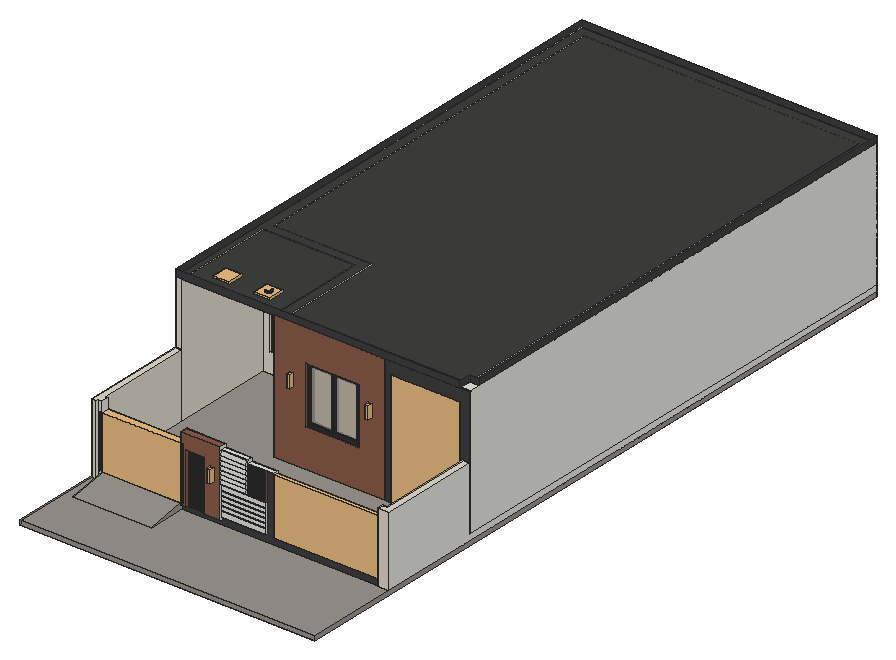
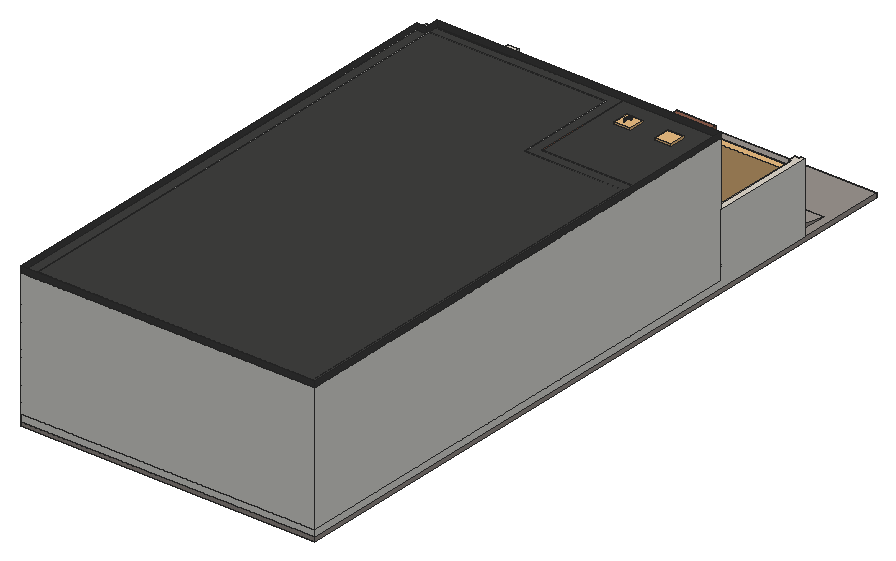
# SketchUp Ruby script. Lengths in inches.
U = 1.inch
M = Sketchup.active_model
def pt(a) = Geom::Point3d.new(a.map { |v| v * U })
def face(e, loops, mat)
  f = e.add_face(loops[0].map { |a| pt(a) })
  loops[1..].each { |l| e.add_face(l.map { |a| pt(a) }).erase! }
  f.material = f.back_material = mat if mat
  f
end
# faces: each face lists its corners as indices into pts; further lists are holes
def faces(e, pts, list, mat = nil) = list.each { |f| face(e, (f[0].is_a?(Array) ? f : [f]).map { |l| l.map { |i| pts[i] } }, mat) }
# xy, xz, yz: faces in a plane at the given z, y or x. An outline is a flat list of corners, or four numbers for a rectangle; further outlines are holes
def ring(l) = l.size == 4 ? [[l[0], l[1]], [l[2], l[1]], [l[2], l[3]], [l[0], l[3]]] : l.each_slice(2).to_a
def flat(e, list, mat, &to3) = list.each { |f| face(e, (f[0].is_a?(Array) ? f : [f]).map { |l| ring(l).map { |u, v| to3.(u, v) } }, mat) }
def xy(e, z, list, mat = nil) = flat(e, list, mat) { |x, y| [x, y, z] }
def xz(e, y, list, mat = nil) = flat(e, list, mat) { |x, z| [x, y, z] }
def yz(e, x, list, mat = nil) = flat(e, list, mat) { |y, z| [x, y, z] }
def lines(e, pts, list) = list.each { |a, b| e.add_line(pt(pts[a]), pt(pts[b])) }
# prism: a flat outline (further loops are holes) pulled along v
def prism(e, loops, v, mat = nil)
  f = face(e, loops, mat); d = Geom::Vector3d.new(v.map { |x| x * U })
  f.pushpull(f.normal.samedirection?(d) ? d.length : -d.length)
end
def box(e, o, s, mat = nil) = prism(e, [[o, [o[0] + s[0], o[1], o[2]], [o[0] + s[0], o[1] + s[1], o[2]], [o[0], o[1] + s[1], o[2]]]], [0, 0, s[2]], mat)
def at(x, y, z, deg = 0) = Geom::Transformation.translation(pt([x, y, z])) * Geom::Transformation.rotation(ORIGIN, Z_AXIS, deg.degrees)
def axes(o, x, y, z) = Geom::Transformation.new([*x, 0, *y, 0, *z, 0, *pt(o).to_a, 1])
def part(name) = M.definitions.add(name)
# library, detail: a bought-in or finely detailed component or shape, given as its bounding box
def library(name, o, s) = part(name).tap { |d| box(d.entities, o, s) }
def detail(e, o, s) = box(e.add_group.entities, o, s)
def put(e, d, t, mat = nil) = e.add_instance(d, t).tap { |i| i.material = mat if mat }
def group(e, t, mat = nil) = e.add_group.tap { |g| g.transformation = t; g.material = mat if mat }.entities
root = M.entities
M.materials.add("1448 AP 8253 RAVEN SONG").color = [64, 64, 63]
M.materials.add("[Chris_Hair]").color = [71, 76, 74]
M.materials.add("[Granite Tile]").color = [155, 148, 143]
M.materials.add("[Steel Brushed Stainless]").color = [51, 51, 51]
M.materials.add("[Stone Vein Gray]").color = [63, 63, 63]
M.materials.add("[Tile Various Tan]").color = [223, 216, 204]
M.materials.add("[Translucent Glass Gray]").color = [181, 181, 181]
M.materials["[Translucent Glass Gray]"].alpha = 0.5
M.materials.add("[Wax 02]").color = [139, 92, 74]
M.materials.add("[Wood Veneer 01]").color = [91, 58, 35]
c1 = part("8")
box(c1.entities,[0,0.25,0],[0.5,0.25,24.5])
c2 = part("9")
box(c2.entities,[0,0,0],[0.25,0.25,48.1875])
c3 = library("Group\#151",[0,0,0],[124.17,4.81,62])
c4 = library("Curtains",[0,0,0],[121.73,8.19,117.22])
c5 = library("porte moderne noir",[57.21,0.32,0],[43.81,4.72,87.03])
c6 = part("Group\#3")
g1 = group(c6.entities,at(0,3,0))
prism(g1,[[[9,0,0],[0,0,0],[0,0,72],[9,0,72]],[[0.75,0,71.25],[0.75,0,0.75],[8.25,0,0.75],[8.25,0,71.25]]],[0,-1,0])
g2 = group(g1,at(0.75,-0.26,0.75),"[Translucent Glass Gray]")
box(g2,[0,-0.47,0],[7.5,0.47,70.5])
c7 = part("Group\#8")
g3 = group(c7.entities,at(0,1.75,0))
prism(g3,[[[21,0,0],[0,0,0],[0,0,50],[21,0,50]],[[20,0,49],[1,0,49],[1,0,1],[20,0,1]]],[0,-1.5,0])
g4 = group(g3,at(1,-0.5,1),"[Translucent Glass Gray]")
box(g4,[0,-0.47,0],[19,0.47,48])
c8 = library("Group\#93",[0,-4.51,0],[63,7.09,108])
c9 = library("Component",[1.03,-1.63,0],[72.41,6.81,50.39])
c10 = library("WALL LIGHT 69",[4.19,4.05,-8.78],[4.61,5.7,17.13])
c11 = library("11",[-5.64,-5.64,-13.23],[15.28,15.28,13.23])
xy(root,120,[[[9.27,183,9.27,663,287.37,663,287.37,195,278.1,195,278.1,183],[39.35,204,39.59,204,39.66,204.01,39.74,204.01,39.9,204.03,39.98,204.05,40.05,204.0625,40.13,204.08,40.21,204.1,40.28,204.12,40.36,204.14,40.43,204.17,40.51,204.19,40.72,204.28,40.79,204.32,40.86,204.35,41.07,204.47,41.13,204.52,41.2,204.5625,41.26,204.61,41.56,204.86,41.61,204.92,41.67,204.98,41.82,205.16,41.86,205.22,41.91,205.28,41.95,205.35,42,205.42,42.04,205.48,42.08,205.55,42.11,205.62,42.15,205.69,42.21,205.83,42.24,205.91,42.3,206.05,42.32,206.13,42.34,206.2,42.38,206.36,42.4,206.43,42.43,206.67,42.4375,206.74,42.44,206.82,42.45,206.9,42.45,207.14,42.44,207.21,42.4375,207.29,42.43,207.37,42.42,207.45,42.4,207.53,42.39,207.6,42.35,207.76,42.33,207.83,42.31,207.91,42.28,207.98,42.26,208.06,42.17,208.27,42.13,208.34,42.1,208.41,41.98,208.62,41.93,208.68,41.89,208.75,41.59,209.11,41.53,209.16,41.47,209.22,41.29,209.37,41.23,209.41,41.17,209.46,41.1,209.5,41.03,209.55,40.97,209.59,40.83,209.66,40.76,209.7,40.6875,209.73,40.62,209.76,40.54,209.79,40.4,209.85,40.32,209.87,40.25,209.89,40.09,209.93,40.02,209.95,39.78,209.98,39.71,209.99,39.63,209.99,39.55,210,39.3125,210,39.24,209.99,39.16,209.99,39,209.97,38.92,209.95,38.85,209.9375,38.77,209.92,38.69,209.9,38.62,209.88,38.54,209.86,38.47,209.83,38.39,209.81,38.18,209.72,38.11,209.68,38.04,209.65,37.83,209.53,37.77,209.48,37.7,209.4375,37.64,209.39,37.34,209.14,37.29,209.08,37.23,209.02,37.08,208.84,37.04,208.78,36.99,208.72,36.95,208.65,36.9,208.58,36.86,208.52,36.82,208.45,36.79,208.38,36.75,208.31,36.72,208.24,36.6875,208.17,36.66,208.09,36.6,207.95,36.58,207.87,36.56,207.8,36.52,207.64,36.5,207.57,36.47,207.33,36.46,207.26,36.46,207.18,36.45,207.1,36.45,206.86,36.46,206.79,36.46,206.71,36.48,206.55,36.5,206.47,36.51,206.4,36.55,206.24,36.57,206.17,36.59,206.09,36.62,206.02,36.64,205.94,36.73,205.73,36.77,205.66,36.8,205.59,36.92,205.38,36.97,205.32,37.01,205.25,37.26,204.95,37.3125,204.89,37.37,204.84,37.43,204.78,37.61,204.63,37.67,204.59,37.73,204.54,37.8,204.5,37.87,204.45,37.93,204.41,38.07,204.34,38.14,204.3,38.28,204.24,38.36,204.21,38.5,204.15,38.58,204.13,38.65,204.11,38.81,204.07,38.88,204.05,39.12,204.02,39.19,204.01,39.27,204.01],[77.87,204,78.11,204,78.18,204.01,78.26,204.01,78.42,204.03,78.5,204.05,78.57,204.0625,78.65,204.08,78.73,204.1,78.8,204.12,78.88,204.14,78.95,204.17,79.03,204.19,79.24,204.28,79.3125,204.32,79.38,204.35,79.59,204.47,79.65,204.52,79.72,204.5625,79.78,204.61,80.08,204.86,80.13,204.92,80.1875,204.98,80.24,205.04,80.34,205.16,80.38,205.22,80.43,205.28,80.47,205.35,80.52,205.42,80.56,205.48,80.6,205.55,80.63,205.62,80.67,205.69,80.73,205.83,80.76,205.91,80.82,206.05,80.84,206.13,80.86,206.2,80.9,206.36,80.92,206.43,80.95,206.67,80.96,206.74,80.96,206.82,80.97,206.9,80.97,207.14,80.96,207.21,80.96,207.29,80.95,207.37,80.9375,207.45,80.92,207.53,80.91,207.6,80.89,207.68,80.875,207.76,80.85,207.83,80.83,207.91,80.8,207.98,80.78,208.06,80.72,208.2,80.6875,208.27,80.65,208.34,80.62,208.41,80.5,208.62,80.45,208.68,80.41,208.75,80.36,208.81,80.3125,208.87,80.26,208.93,80.11,209.11,80.05,209.16,79.99,209.22,79.93,209.27,79.875,209.32,79.8125,209.37,79.75,209.41,79.6875,209.46,79.62,209.5,79.55,209.55,79.49,209.59,79.35,209.66,79.28,209.7,79.14,209.76,79.0625,209.79,78.99,209.82,78.92,209.85,78.84,209.87,78.77,209.89,78.61,209.93,78.54,209.95,78.3,209.98,78.23,209.99,78.15,209.99,78.07,210,77.83,210,77.76,209.99,77.68,209.99,77.52,209.97,77.44,209.95,77.37,209.9375,77.29,209.92,77.21,209.9,77.14,209.88,77.0625,209.86,76.99,209.83,76.91,209.81,76.7,209.72,76.625,209.68,76.56,209.65,76.35,209.53,76.29,209.48,76.22,209.4375,76.16,209.39,75.86,209.14,75.81,209.08,75.75,209.02,75.6,208.84,75.56,208.78,75.51,208.72,75.47,208.65,75.42,208.58,75.38,208.52,75.34,208.45,75.31,208.38,75.27,208.31,75.21,208.17,75.18,208.09,75.15,208.02,75.125,207.95,75.1,207.87,75.08,207.8,75.04,207.64,75.02,207.57,74.99,207.33,74.98,207.26,74.98,207.18,74.97,207.1,74.97,206.86,74.98,206.79,74.98,206.71,75,206.55,75.02,206.47,75.03,206.4,75.07,206.24,75.09,206.17,75.11,206.09,75.14,206.02,75.16,205.94,75.25,205.73,75.29,205.66,75.32,205.59,75.44,205.38,75.49,205.32,75.53,205.25,75.58,205.19,75.625,205.13,75.68,205.07,75.83,204.89,75.89,204.84,75.95,204.78,76.13,204.63,76.19,204.59,76.25,204.54,76.32,204.5,76.39,204.45,76.45,204.41,76.59,204.34,76.66,204.3,76.8,204.24,76.95,204.18,77.02,204.15,77.1,204.13,77.17,204.11,77.33,204.07,77.4,204.05,77.64,204.02,77.71,204.01,77.79,204.01]]],"1448 AP 8253 RAVEN SONG")
xz(root,183,[[9.27,120,278.1,126]],"1448 AP 8253 RAVEN SONG")
xz(root,195,[[278.1,120,287.37,126]],"1448 AP 8253 RAVEN SONG")
xz(root,204,[[77.87,120,77.95,123],[77.95,120,78.03,123],[78.03,120,78.11,123]],"1448 AP 8253 RAVEN SONG")
xz(root,204.01,[[77.71,120,77.79,123],[78.18,120,78.26,123]],"1448 AP 8253 RAVEN SONG")
xz(root,663,[[9.27,120,287.37,126]],"1448 AP 8253 RAVEN SONG")
yz(root,9.27,[[183,120,663,126]],"1448 AP 8253 RAVEN SONG")
yz(root,80.96,[[206.74,120,206.82,123],[207.21,120,207.29,123]],"1448 AP 8253 RAVEN SONG")
yz(root,80.97,[[206.9,120,206.98,123],[206.98,120,207.06,123],[207.06,120,207.14,123]],"1448 AP 8253 RAVEN SONG")
yz(root,278.1,[[183,120,195,126]],"1448 AP 8253 RAVEN SONG")
yz(root,287.37,[[195,120,663,126]],"1448 AP 8253 RAVEN SONG")
p = [[77.48,204.04,120],[77.4,204.05,120],[77.4,204.05,123],[77.48,204.04,123],[77.56,204.03,120],[77.56,204.03,123],
  [77.71,204.01,120],[77.64,204.02,120],[77.64,204.02,123],[77.71,204.01,123],[77.87,204,120],[77.79,204.01,120],
  [77.79,204.01,123],[77.87,204,123],[78.18,204.01,120],[78.11,204,120],[78.11,204,123],[78.18,204.01,123],
  [78.42,204.03,120],[78.34,204.02,120],[78.34,204.02,123],[78.42,204.03,123],[78.26,204.01,120],[78.26,204.01,123],
  [78.5,204.05,120],[78.5,204.05,123],[78.57,204.0625,120],[78.57,204.0625,123],[77.1,204.13,120],[77.02,204.15,120],
  [77.02,204.15,123],[77.1,204.13,123],[77.17,204.11,120],[77.17,204.11,123],[77.33,204.07,120],[77.25,204.09,120],
  [77.25,204.09,123],[77.33,204.07,123],[78.65,204.08,120],[78.65,204.08,123],[78.8,204.12,120],[78.73,204.1,120],
  [78.73,204.1,123],[78.8,204.12,123],[78.88,204.14,120],[78.88,204.14,123],[78.95,204.17,120],[78.95,204.17,123],
  [76.875,204.21,120],[76.8,204.24,120],[76.8,204.24,123],[76.875,204.21,123],[76.95,204.18,120],[76.95,204.18,123],
  [79.1,204.22,120],[79.03,204.19,120],[79.03,204.19,123],[79.1,204.22,123],[79.17,204.25,120],[79.17,204.25,123],
  [79.3125,204.32,120],[79.24,204.28,120],[79.24,204.28,123],[79.3125,204.32,123],[79.38,204.35,120],[79.38,204.35,123],
  [79.45,204.39,120],[79.45,204.39,123],[79.59,204.47,120],[79.52,204.43,120],[79.52,204.43,123],[79.59,204.47,123],
  [79.65,204.52,120],[79.65,204.52,123],[79.72,204.5625,120],[79.72,204.5625,123],[79.78,204.61,120],[79.78,204.61,123],
  [79.84,204.66,120],[79.84,204.66,123],[79.9,204.71,120],[79.9,204.71,123],[79.96,204.76,120],[79.96,204.76,123],
  [80.08,204.86,120],[80.02,204.81,120],[80.02,204.81,123],[80.08,204.86,123],[80.1875,204.98,120],[80.13,204.92,120],
  [80.13,204.92,123],[80.1875,204.98,123],[80.29,205.1,120],[80.24,205.04,120],[80.24,205.04,123],[80.29,205.1,123],
  [80.34,205.16,120],[80.34,205.16,123],[80.38,205.22,120],[80.38,205.22,123],[80.43,205.28,120],[80.43,205.28,123],
  [80.47,205.35,120],[80.47,205.35,123],[80.52,205.42,120],[80.52,205.42,123],[80.56,205.48,120],[80.56,205.48,123],
  [80.6,205.55,120],[80.6,205.55,123],[80.67,205.69,120],[80.63,205.62,120],[80.63,205.62,123],[80.67,205.69,123],
  [80.7,205.76,120],[80.7,205.76,123],[80.76,205.91,120],[80.73,205.83,120],[80.73,205.83,123],[80.76,205.91,123],
  [80.79,205.98,120],[80.79,205.98,123],[80.82,206.05,120],[80.82,206.05,123],[80.86,206.2,120],[80.84,206.13,120],
  [80.84,206.13,123],[80.86,206.2,123],[80.88,206.28,120],[80.88,206.28,123],[80.9,206.36,120],[80.9,206.36,123],
  [80.93,206.51,120],[80.92,206.43,120],[80.92,206.43,123],[80.93,206.51,123],[80.94,206.59,120],[80.94,206.59,123],
  [80.95,206.67,120],[80.95,206.67,123],[80.96,206.74,120],[80.96,206.74,123],[80.97,206.9,120],[80.96,206.82,120],
  [80.96,206.82,123],[80.97,206.9,123],[80.96,207.21,120],[80.97,207.14,120],[80.97,207.14,123],[80.96,207.21,123],
  [80.95,207.37,120],[80.96,207.29,120],[80.96,207.29,123],[80.95,207.37,123],[80.92,207.53,120],[80.9375,207.45,120],
  [80.9375,207.45,123],[80.92,207.53,123],[80.91,207.6,120],[80.91,207.6,123],[80.89,207.68,120],[80.89,207.68,123],
  [80.875,207.76,120],[80.875,207.76,123],[80.83,207.91,120],[80.85,207.83,120],[80.85,207.83,123],[80.83,207.91,123],
  [80.8,207.98,120],[80.8,207.98,123],[80.78,208.06,120],[80.78,208.06,123],[80.72,208.2,120],[80.75,208.13,120],
  [80.75,208.13,123],[80.72,208.2,123],[80.6875,208.27,120],[80.6875,208.27,123],[80.62,208.41,120],[80.65,208.34,120],
  [80.65,208.34,123],[80.62,208.41,123],[80.58,208.48,120],[80.58,208.48,123],[80.5,208.62,120],[80.54,208.55,120],
  [80.54,208.55,123],[80.5,208.62,123],[80.45,208.68,120],[80.45,208.68,123],[80.36,208.81,120],[80.41,208.75,120],
  [80.41,208.75,123],[80.36,208.81,123],[80.3125,208.87,120],[80.3125,208.87,123],[80.21,208.99,120],[80.26,208.93,120],
  [80.26,208.93,123],[80.21,208.99,123],[80.16,209.05,120],[80.16,209.05,123],[80.05,209.16,120],[80.11,209.11,120],
  [80.11,209.11,123],[80.05,209.16,123],[79.93,209.27,120],[79.99,209.22,120],[79.99,209.22,123],[79.93,209.27,123],
  [79.8125,209.37,120],[79.875,209.32,120],[79.875,209.32,123],[79.8125,209.37,123],[79.75,209.41,120],[79.75,209.41,123]]
faces(root,p,[[0,1,2,3],[4,0,3,5],[6,7,8,9],[7,4,5,8],[10,11,12,13],[14,15,16,17],[18,19,20,21],[19,22,23,20],
  [24,18,21,25],[26,24,25,27],[28,29,30,31],[32,28,31,33],[34,35,36,37],[35,32,33,36],[1,34,37,2],[38,26,27,39],
  [40,41,42,43],[41,38,39,42],[44,40,43,45],[46,44,45,47],[48,49,50,51],[29,52,53,30],[52,48,51,53],[54,55,56,57],
  [55,46,47,56],[58,54,57,59],[60,61,62,63],[61,58,59,62],[64,60,63,65],[66,64,65,67],[68,69,70,71],[69,66,67,70],
  [72,68,71,73],[74,72,73,75],[76,74,75,77],[78,76,77,79],[80,78,79,81],[82,80,81,83],[84,85,86,87],[85,82,83,86],
  [88,89,90,91],[89,84,87,90],[92,93,94,95],[93,88,91,94],[96,92,95,97],[98,96,97,99],[100,98,99,101],[102,100,101,103],
  [104,102,103,105],[106,104,105,107],[108,106,107,109],[110,111,112,113],[111,108,109,112],[114,110,113,115],[116,117,118,119],[117,114,115,118],
  [120,116,119,121],[122,120,121,123],[124,125,126,127],[125,122,123,126],[128,124,127,129],[130,128,129,131],[132,133,134,135],[133,130,131,134],
  [136,132,135,137],[138,136,137,139],[140,138,139,141],[142,143,144,145],[146,147,148,149],[150,151,152,153],[154,155,156,157],[155,150,153,156],
  [158,154,157,159],[160,158,159,161],[162,160,161,163],[164,165,166,167],[165,162,163,166],[168,164,167,169],[170,168,169,171],[172,173,174,175],
  [173,170,171,174],[176,172,175,177],[178,179,180,181],[179,176,177,180],[182,178,181,183],[184,185,186,187],[185,182,183,186],[188,184,187,189],
  [190,191,192,193],[191,188,189,192],[194,190,193,195],[196,197,198,199],[197,194,195,198],[200,196,199,201],[202,203,204,205],[203,200,201,204],
  [206,207,208,209],[207,202,205,208],[210,211,212,213],[211,206,209,212],[214,210,213,215]],"1448 AP 8253 RAVEN SONG")
g5 = group(root,at(9.27,84,-6),"[Granite Tile]")
box(g5,[0,-84,-4],[278.1,663,4])
g6 = group(root,at(9.27,183,0))
xy(g6,-6,[[0,-99,0,480,278.1,480,278.1,-96,267.8,-96,267.8,-95,8.24,-95,8.24,-97,4.12,-97,4.12,-99]])
xy(g6,-2,[[82.4,-96.5,87.55,-95],[104.03,-96.5,119.48,-95],[87.55,-95,104.03,-95,104.03,-94,87.81,-94,87.81,-94.25,87.55,-94.25]])
xy(g6,0,[[8.24,-95,82.4,-95,82.4,-90,168.92,-90,168.92,-95,267.8,-95,267.8,-90,271.92,-90,271.92,0,278.1,0,278.1,480,0,480,0,0,6.18,0,6.18,-90,8.24,-90]],"[Granite Tile]")
xy(g6,1,[[119.48,-96,162.74,-95]])
xy(g6,6,[[119.48,-96,162.74,-95.75]])
xy(g6,6.25,[[119.48,-96,162.74,-95.75]])
xy(g6,10.25,[[119.48,-96,162.74,-95.75]])
xy(g6,10.5,[[119.48,-96,162.74,-95.75]])
xy(g6,14.5,[[119.48,-96,162.74,-95.75]])
xy(g6,14.75,[[119.48,-96,162.74,-95.75]])
xy(g6,18.75,[[119.48,-96,162.74,-95.75]])
xy(g6,19,[[119.48,-96,162.74,-95.75]])
xy(g6,23,[[119.48,-96,162.74,-95.75]])
xy(g6,23.25,[[119.48,-96,162.74,-95.75]])
xy(g6,27.75,[[119.48,-96,144.2,-95],[144.2,-96,162.74,-95]])
xy(g6,46,[[87.55,-96.5,104.03,-94]],"[Wax 02]")
xy(g6,54,[[144.2,-95,168.92,-90]])
xy(g6,57,[[119.48,-95,144.2,-90]])
xy(g6,60,[[0,-99,4.12,-99,4.12,-97,8.24,-97,8.24,-90,6.18,-90,6.18,0,0,0],[267.8,-96,278.1,-96,278.1,0,271.92,0,271.92,-90,267.8,-90]],"[Tile Various Tan]")
xy(g6,60,[[82.4,-96.5,119.48,-90]],"[Wax 02]")
xz(g6,-99,[[0,-6,4.12,60]],"[Tile Various Tan]")
xz(g6,-97,[[4.12,-6,8.24,60]],"[Tile Various Tan]")
xz(g6,-96.5,[[82.4,-2,87.55,-2,87.55,46,104.03,46,104.03,-2,119.48,-2,119.48,60,82.4,60]],"[Wax 02]")
xz(g6,-96,[[119.48,1,162.74,6],[119.48,6.25,162.74,10.25],[119.48,10.5,162.74,14.5],[119.48,14.75,162.74,18.75],[119.48,19,162.74,23],
  [119.48,23.25,162.74,27.75]])
xz(g6,-96,[[267.8,-6,278.1,60]],"[Tile Various Tan]")
xz(g6,-95.75,[[119.48,6,162.74,6.25],[119.48,10.25,162.74,10.5],[119.48,14.5,162.74,14.75],[119.48,18.75,162.74,19],[119.48,23,162.74,23.25]])
xz(g6,-95,[[119.48,28,144.2,57],[144.2,28,162.74,54]])
xz(g6,-95,[[82.4,-6,267.8,-6,267.8,0,168.92,0,168.92,54,162.74,54,162.74,28,119.48,28,119.48,27.75,162.74,27.75,162.74,1,119.48,1,119.48,-2,82.4,-2]],"1448 AP 8253 RAVEN SONG")
xz(g6,-94,[[87.55,-2,104.03,46]])
xz(g6,-90,[[6.18,0,8.24,60],[82.4,0,82.4,60,119.48,60,119.48,57,144.2,57,144.2,54,168.92,54,168.92,0],[267.8,0,271.92,60]])
xz(g6,0,[[0,0,6.18,60],[271.92,0,278.1,60]])
xz(g6,480,[[0,-6,278.1,0]])
yz(g6,0,[[-99,-6,-99,60,0,60,0,0,480,0,480,-6]])
yz(g6,4.12,[[-99,-6,-97,60]])
yz(g6,6.18,[[-90,0,0,60]],"[Tile Various Tan]")
yz(g6,8.24,[[-97,-6,-95,-6,-95,0,-90,0,-90,60,-97,60]])
yz(g6,82.4,[[-96.5,-2,-96.5,60,-90,60,-90,0,-95,0,-95,-2]],"[Wax 02]")
yz(g6,87.55,[[-96.5,-2,-94,46]],"[Wax 02]")
yz(g6,104.03,[[-96.5,-2,-94,46]],"[Wax 02]")
yz(g6,119.48,[[-96.5,-2,-95,-2,-95,1,-96,1,-96,6,-95.75,6,-95.75,6.25,-96,6.25,-96,10.25,-95.75,10.25,-95.75,10.5,-96,10.5,-96,14.5,-95.75,14.5,-95.75,14.75,-96,14.75,-96,18.75,-95.75,18.75,-95.75,19,-96,19,-96,23,-95.75,23,-95.75,23.25,-96,23.25,-96,27.75,-95,27.75,-95,57,-96.5,57],[-96.5,57,-90,60]])
yz(g6,144.2,[[-95,54,-90,57]])
yz(g6,162.74,[[-96,1,-95,1,-95,27.75,-96,27.75,-96,23.25,-95.75,23.25,-95.75,23,-96,23,-96,19,-95.75,19,-95.75,18.75,-96,18.75,-96,14.75,-95.75,14.75,-95.75,14.5,-96,14.5,-96,10.5,-95.75,10.5,-95.75,10.25,-96,10.25,-96,6.25,-95.75,6.25,-95.75,6,-96,6]])
yz(g6,168.92,[[-95,0,-90,54]])
yz(g6,267.8,[[-96,-6,-96,60,-90,60,-90,0,-95,0,-95,-6]])
yz(g6,271.92,[[-90,0,0,60]],"[Tile Various Tan]")
yz(g6,278.1,[[-96,-6,480,-6,480,0,0,0,0,60,-96,60]])
g7 = group(g6,at(144.2,-96,28),"[Wax 02]")
xy(g7,0,[[0,0,18.54,1]])
xy(g7,0.75,[[0.77,0,17.77,0.8]])
xy(g7,25.25,[[0.77,0,17.77,0.8]])
xy(g7,26,[[0,0,18.54,1]])
xz(g7,0,[[[0,0,18.54,26],[0.77,0.75,17.77,25.25]]])
xz(g7,0.8,[[0.77,0.75,17.77,25.25]])
xz(g7,1,[[0,0,18.54,26]])
yz(g7,0,[[0,0,1,26]])
yz(g7,0.77,[[0,0.75,0.8,25.25]])
yz(g7,17.77,[[0,0.75,0.8,25.25]])
yz(g7,18.54,[[0,0,1,26]])
put(g7,c1,axes([16.74,0.2,0.75],[1.03,0,0],[0,0.8,0],[0,0,1]))
put(g7,c1,axes([15.71,0.2,0.75],[1.03,0,0],[0,0.8,0],[0,0,1]))
put(g7,c1,axes([11.59,0.2,0.75],[1.03,0,0],[0,0.8,0],[0,0,1]))
put(g7,c1,axes([10.56,0.2,0.75],[1.03,0,0],[0,0.8,0],[0,0,1]))
put(g7,c1,axes([12.62,0.2,0.75],[1.03,0,0],[0,0.8,0],[0,0,1]))
put(g7,c1,axes([9.53,0.2,0.75],[1.03,0,0],[0,0.8,0],[0,0,1]))
put(g7,c1,axes([8.5,0.2,0.75],[1.03,0,0],[0,0.8,0],[0,0,1]))
put(g7,c1,axes([7.47,0.2,0.75],[1.03,0,0],[0,0.8,0],[0,0,1]))
put(g7,c1,axes([5.41,0.2,0.75],[1.03,0,0],[0,0.8,0],[0,0,1]))
put(g7,c1,axes([6.4375,0.2,0.75],[1.03,0,0],[0,0.8,0],[0,0,1]))
put(g7,c1,axes([4.38,0.2,0.75],[1.03,0,0],[0,0.8,0],[0,0,1]))
put(g7,c1,axes([2.32,0.2,0.75],[1.03,0,0],[0,0.8,0],[0,0,1]))
put(g7,c1,axes([3.35,0.2,0.75],[1.03,0,0],[0,0.8,0],[0,0,1]))
put(g7,c1,axes([13.65,0.2,0.75],[1.03,0,0],[0,0.8,0],[0,0,1]))
put(g7,c1,axes([14.68,0.2,0.75],[1.03,0,0],[0,0.8,0],[0,0,1]))
put(g7,c1,axes([1.29,0.2,0.75],[1.03,0,0],[0,0.8,0],[0,0,1]))
g8 = group(g6,at(119.48,-95,28))
prism(g8,[[[0,0,29],[0,0,0],[0,-1,0],[0,-1,1],[0,-1.5,1],[0,-1,5],[0,-1.5,5],[0,-1,9],[0,-1.5,9],[0,-1,13],[0,-1.5,13],[0,-1,17],[0,-1.5,17],[0,-1,21],[0,-1.5,21],[0,-1,25],[0,-1.5,25],[0,-1,29]]],[24.72,0,0])
g9 = group(g6,at(87.55,-94.25,-2),"[Wax 02]")
put(g9,c2,axes([0.32,0,0],[1.03,0,0],[0,1,0],[0,0,1]))
put(g9,c2,axes([15.25,0,0],[1.03,0,0],[0,1,0],[0,0,1]))
put(g9,c2,axes([12.98,0,0],[1.03,0,0],[0,1,0],[0,0,1]))
put(g9,c2,axes([13.3,0,0],[1.03,0,0],[0,1,0],[0,0,1]))
put(g9,c2,axes([12.33,0,0],[1.03,0,0],[0,1,0],[0,0,1]))
put(g9,c2,axes([14.28,0,0],[1.03,0,0],[0,1,0],[0,0,1]))
put(g9,c2,axes([12,0,0],[1.03,0,0],[0,1,0],[0,0,1]))
put(g9,c2,axes([13.95,0,0],[1.03,0,0],[0,1,0],[0,0,1]))
put(g9,c2,axes([11.36,0,0],[1.03,0,0],[0,1,0],[0,0,1]))
put(g9,c2,axes([15.9,0,0],[1.03,0,0],[0,1,0],[0,0,1]))
put(g9,c2,axes([14.92,0,0],[1.03,0,0],[0,1,0],[0,0,1]))
put(g9,c2,axes([13.625,0,0],[1.03,0,0],[0,1,0],[0,0,1]))
put(g9,c2,axes([11.68,0,0],[1.03,0,0],[0,1,0],[0,0,1]))
put(g9,c2,axes([12.65,0,0],[1.03,0,0],[0,1,0],[0,0,1]))
put(g9,c2,axes([15.57,0,0],[1.03,0,0],[0,1,0],[0,0,1]))
put(g9,c2,axes([14.6,0,0],[1.03,0,0],[0,1,0],[0,0,1]))
put(g9,c2,axes([5.84,0,0],[1.03,0,0],[0,1,0],[0,0,1]))
put(g9,c2,axes([0,0,0],[1.03,0,0],[0,1,0],[0,0,1]))
put(g9,c2,axes([9.41,0,0],[1.03,0,0],[0,1,0],[0,0,1]))
put(g9,c2,axes([8.11,0,0],[1.03,0,0],[0,1,0],[0,0,1]))
put(g9,c2,axes([8.76,0,0],[1.03,0,0],[0,1,0],[0,0,1]))
put(g9,c2,axes([8.4375,0,0],[1.03,0,0],[0,1,0],[0,0,1]))
put(g9,c2,axes([6.16,0,0],[1.03,0,0],[0,1,0],[0,0,1]))
put(g9,c2,axes([16.22,0,0],[1.03,0,0],[0,1,0],[0,0,1]))
put(g9,c2,axes([9.08,0,0],[1.03,0,0],[0,1,0],[0,0,1]))
put(g9,c2,axes([7.79,0,0],[1.03,0,0],[0,1,0],[0,0,1]))
put(g9,c2,axes([9.73,0,0],[1.03,0,0],[0,1,0],[0,0,1]))
put(g9,c2,axes([10.06,0,0],[1.03,0,0],[0,1,0],[0,0,1]))
put(g9,c2,axes([10.71,0,0],[1.03,0,0],[0,1,0],[0,0,1]))
put(g9,c2,axes([10.38,0,0],[1.03,0,0],[0,1,0],[0,0,1]))
put(g9,c2,axes([6.49,0,0],[1.03,0,0],[0,1,0],[0,0,1]))
put(g9,c2,axes([6.8125,0,0],[1.03,0,0],[0,1,0],[0,0,1]))
put(g9,c2,axes([7.14,0,0],[1.03,0,0],[0,1,0],[0,0,1]))
put(g9,c2,axes([7.46,0,0],[1.03,0,0],[0,1,0],[0,0,1]))
put(g9,c2,axes([5.52,0,0],[1.03,0,0],[0,1,0],[0,0,1]))
put(g9,c2,axes([4.87,0,0],[1.03,0,0],[0,1,0],[0,0,1]))
put(g9,c2,axes([0.65,0,0],[1.03,0,0],[0,1,0],[0,0,1]))
put(g9,c2,axes([5.19,0,0],[1.03,0,0],[0,1,0],[0,0,1]))
put(g9,c2,axes([1.3,0,0],[1.03,0,0],[0,1,0],[0,0,1]))
put(g9,c2,axes([2.6,0,0],[1.03,0,0],[0,1,0],[0,0,1]))
put(g9,c2,axes([4.22,0,0],[1.03,0,0],[0,1,0],[0,0,1]))
put(g9,c2,axes([11.03,0,0],[1.03,0,0],[0,1,0],[0,0,1]))
put(g9,c2,axes([1.95,0,0],[1.03,0,0],[0,1,0],[0,0,1]))
put(g9,c2,axes([0.97,0,0],[1.03,0,0],[0,1,0],[0,0,1]))
put(g9,c2,axes([3.57,0,0],[1.03,0,0],[0,1,0],[0,0,1]))
put(g9,c2,axes([2.27,0,0],[1.03,0,0],[0,1,0],[0,0,1]))
put(g9,c2,axes([2.92,0,0],[1.03,0,0],[0,1,0],[0,0,1]))
put(g9,c2,axes([3.24,0,0],[1.03,0,0],[0,1,0],[0,0,1]))
put(g9,c2,axes([1.62,0,0],[1.03,0,0],[0,1,0],[0,0,1]))
put(g9,c2,axes([4.54,0,0],[1.03,0,0],[0,1,0],[0,0,1]))
put(g9,c2,axes([3.89,0,0],[1.03,0,0],[0,1,0],[0,0,1]))
put(g6,c3,axes([168.92,-91.11,0],[0.79635,0,0],[0,-0.81,0],[0,0,0.8586]),"[Chris_Hair]")
g10 = group(g6,at(8.24,-95,-6),"[Granite Tile]")
prism(g10,[[[74.16,0,0],[74.16,0,6],[74.16,-36,0]]],[-74.16,0,0])
put(root,c4,axes([201.66,192,0],[0.62727,0,0],[0,0.7,0],[0,0,0.973]))
g11 = group(root,at(9.27,183,0))
xy(g11,0,[[0,0,0,480,278.1,480,278.1,1,268.83,1,268.83,471,9.27,471,9.27,105,27.81,105,27.81,96,6.18,96,6.18,0],[92.7,0,92.7,96,71.07,96,71.07,105,101.97,105,101.97,9,203.94,9,203.94,1,197.76,1,197.76,0]])
xy(g11,18,[[12.36,96,21.63,105],[77.25,96,86.52,105]])
xy(g11,36,[[123.6,0,173.04,9]],"[Wax 02]")
xy(g11,90,[[12.36,96,21.63,105],[27.81,96,71.07,105],[77.25,96,86.52,105]])
xy(g11,90,[[123.6,0,173.04,9]],"[Wax 02]")
xy(g11,108,[[203.94,1,268.83,9]])
xy(g11,120,[[[0,0,6.18,0,6.18,96,92.7,96,92.7,0,197.76,0,197.76,1,278.1,1,278.1,480,0,480],[101.97,9,101.97,105,9.27,105,9.27,471,268.83,471,268.83,9]]])
xz(g11,0,[[0,0,6.18,120]],"[Tile Various Tan]")
xz(g11,0,[[[92.7,0,197.76,120],[123.6,36,173.04,90]]],"[Wax 02]")
xz(g11,1,[[197.76,0,203.94,0,203.94,108,268.83,108,268.83,0,278.1,0,278.1,120,197.76,120]])
xz(g11,9,[[[101.97,0,101.97,120,268.83,120,268.83,108,203.94,108,203.94,0],[123.6,36,173.04,90]]])
xz(g11,96,[[[6.18,0,27.81,0,27.81,90,71.07,90,71.07,0,92.7,0,92.7,120,6.18,120],[77.25,18,86.52,90],[12.36,18,21.63,90]]],"[Tile Various Tan]")
xz(g11,105,[[[9.27,0,9.27,120,101.97,120,101.97,0,71.07,0,71.07,90,27.81,90,27.81,0],[77.25,18,86.52,90],[12.36,18,21.63,90]]])
xz(g11,471,[[9.27,0,268.83,120]])
xz(g11,480,[[0,0,278.1,120]])
yz(g11,0,[[0,0,480,120]])
yz(g11,6.18,[[0,0,96,120]],"[Tile Various Tan]")
yz(g11,9.27,[[105,0,471,120]])
yz(g11,12.36,[[96,18,105,90]])
yz(g11,21.63,[[96,18,105,90]])
yz(g11,27.81,[[96,0,105,90]])
yz(g11,71.07,[[96,0,105,90]])
yz(g11,77.25,[[96,18,105,90]])
yz(g11,86.52,[[96,18,105,90]])
yz(g11,92.7,[[0,0,96,120]],"[Wax 02]")
yz(g11,101.97,[[9,0,105,120]])
yz(g11,123.6,[[0,36,9,90]],"[Wax 02]")
yz(g11,173.04,[[0,36,9,90]],"[Wax 02]")
yz(g11,197.76,[[0,0,1,120]])
yz(g11,203.94,[[1,0,9,108]])
yz(g11,268.83,[[1,0,9,108],[9,0,471,120]])
yz(g11,278.1,[[1,0,480,120]])
put(g11,c5,axes([-28.67,97.68,0],[0.98737,0,0],[0,1,0],[0,0,1.03407]))
put(g11,c6,axes([12.36,96,18],[1.03,0,0],[0,1,0],[0,0,1]),"[Wood Veneer 01]")
put(g11,c6,axes([77.25,96,18],[1.03,0,0],[0,1,0],[0,0,1]),"[Wood Veneer 01]")
g12 = group(g11,at(123.6,4,36),"[Steel Brushed Stainless]")
g13 = group(g12,at(0,0,0))
prism(g13,[[[49.44,0,0],[0,0,0],[0,0,54],[49.44,0,54]],[[23.69,0,2],[23.69,0,52],[2.06,0,52],[2.06,0,2]],[[25.75,0,2],[47.38,0,2],[47.38,0,52],[25.75,0,52]]],[0,-2,0])
put(g13,c7,axes([2.06,-2,2],[1.03,0,0],[0,1,0],[0,0,1]))
put(g13,c7,axes([25.75,-2,2],[1.03,0,0],[0,1,0],[0,0,1]))
g14 = group(g11,at(197.76,1,0),"[Stone Vein Gray]")
prism(g14,[[[80.34,0,0],[71.07,0,0],[71.07,0,108],[6.18,0,108],[6.18,0,0],[0,0,0],[0,0,120],[80.34,0,120]]],[0,-1,0])
put(g11,c8,axes([203.94,4.51,0],[1.03,0,0],[0,1,0],[0,0,1]),"[Steel Brushed Stainless]")
put(root,c9,axes([14.5,88,0],[1.0816,0,0],[0,1,0],[0,0,1]))
put(root,c4,axes([18.54,288,0],[0.721,0,0],[0,0.7,0],[0,0,0.812]))
put(root,c4,axes([119.41,192,21.49],[0.62727,0,0],[0,0.609,0],[0,0,0.609]))
put(root,c10,axes([116.4375,79.68,34.52],[0.7,0,0],[0,0.7,0],[0,0,0.7]))
put(root,c10,axes([188.3,176.18,71.52],[0.7,0,0],[0,0.7,0],[0,0,0.7]))
put(root,c10,axes([114.55,176.18,71.52],[0.7,0,0],[0,0.7,0],[0,0,0.7]))
put(root,c11,at(37.45,205,121.38))
put(root,c11,at(75.97,205,121.38))
